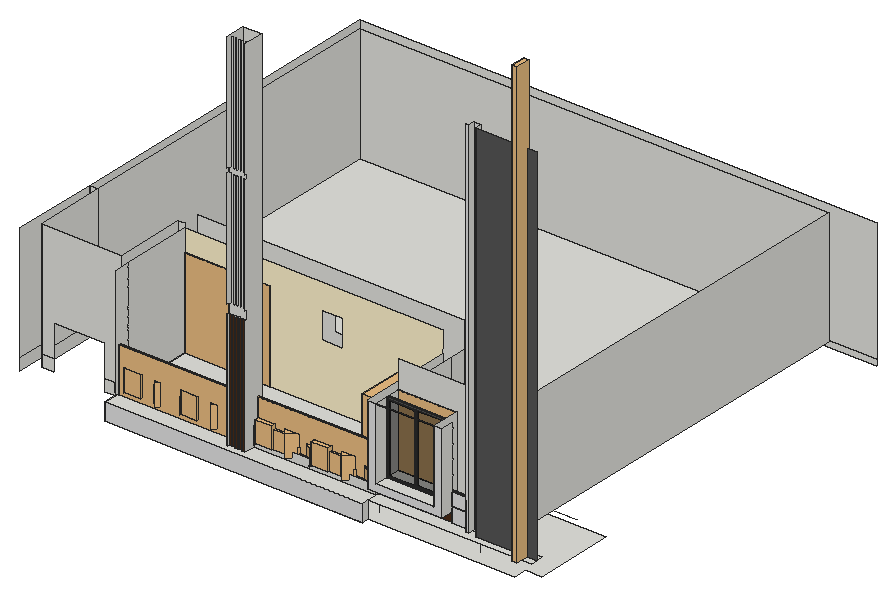
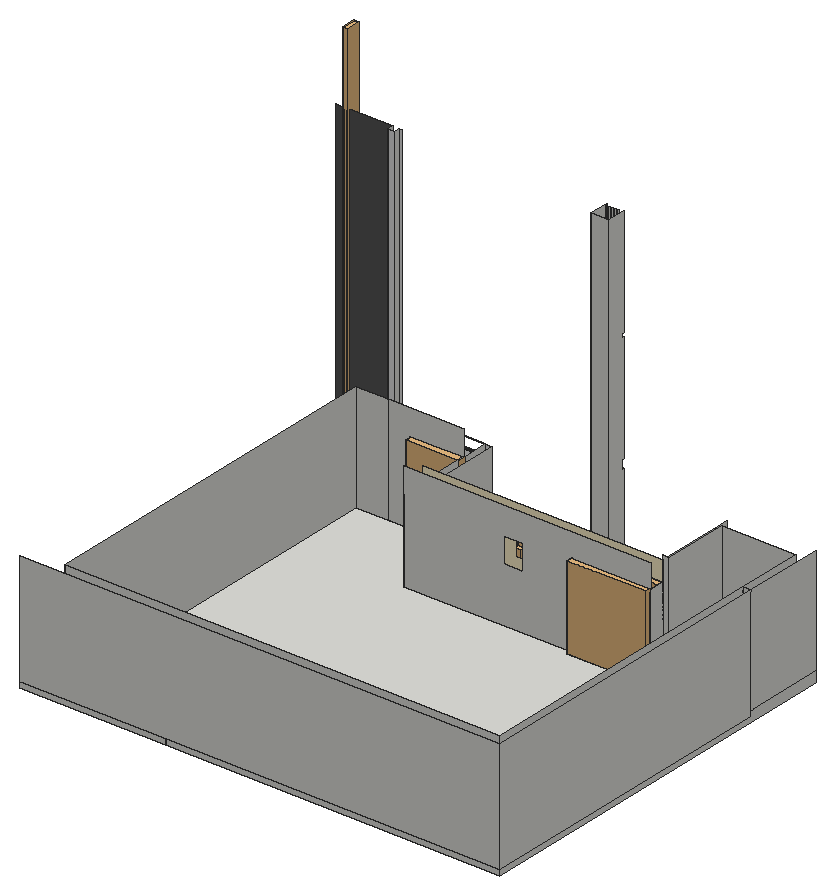
# SketchUp Ruby script. Lengths in inches.
U = 1.inch
M = Sketchup.active_model
def pt(a) = Geom::Point3d.new(a.map { |v| v * U })
def face(e, loops, mat)
  f = e.add_face(loops[0].map { |a| pt(a) })
  loops[1..].each { |l| e.add_face(l.map { |a| pt(a) }).erase! }
  f.material = f.back_material = mat if mat
  f
end
# faces: each face lists its corners as indices into pts; further lists are holes
def faces(e, pts, list, mat = nil) = list.each { |f| face(e, (f[0].is_a?(Array) ? f : [f]).map { |l| l.map { |i| pts[i] } }, mat) }
# xy, xz, yz: faces in a plane at the given z, y or x. An outline is a flat list of corners, or four numbers for a rectangle; further outlines are holes
def ring(l) = l.size == 4 ? [[l[0], l[1]], [l[2], l[1]], [l[2], l[3]], [l[0], l[3]]] : l.each_slice(2).to_a
def flat(e, list, mat, &to3) = list.each { |f| face(e, (f[0].is_a?(Array) ? f : [f]).map { |l| ring(l).map { |u, v| to3.(u, v) } }, mat) }
def xy(e, z, list, mat = nil) = flat(e, list, mat) { |x, y| [x, y, z] }
def xz(e, y, list, mat = nil) = flat(e, list, mat) { |x, z| [x, y, z] }
def yz(e, x, list, mat = nil) = flat(e, list, mat) { |y, z| [x, y, z] }
def lines(e, pts, list) = list.each { |a, b| e.add_line(pt(pts[a]), pt(pts[b])) }
# prism: a flat outline (further loops are holes) pulled along v
def prism(e, loops, v, mat = nil)
  f = face(e, loops, mat); d = Geom::Vector3d.new(v.map { |x| x * U })
  f.pushpull(f.normal.samedirection?(d) ? d.length : -d.length)
end
def box(e, o, s, mat = nil) = prism(e, [[o, [o[0] + s[0], o[1], o[2]], [o[0] + s[0], o[1] + s[1], o[2]], [o[0], o[1] + s[1], o[2]]]], [0, 0, s[2]], mat)
def at(x, y, z, deg = 0) = Geom::Transformation.translation(pt([x, y, z])) * Geom::Transformation.rotation(ORIGIN, Z_AXIS, deg.degrees)
def axes(o, x, y, z) = Geom::Transformation.new([*x, 0, *y, 0, *z, 0, *pt(o).to_a, 1])
def part(name) = M.definitions.add(name)
# library, detail: a bought-in or finely detailed component or shape, given as its bounding box
def library(name, o, s) = part(name).tap { |d| box(d.entities, o, s) }
def detail(e, o, s) = box(e.add_group.entities, o, s)
def put(e, d, t, mat = nil) = e.add_instance(d, t).tap { |i| i.material = mat if mat }
def group(e, t, mat = nil) = e.add_group.tap { |g| g.transformation = t; g.material = mat if mat }.entities
root = M.entities
M.materials.add("Glass_Tinted_Gray").color = [0, 0, 0]
M.materials["Glass_Tinted_Gray"].alpha = 0.125
M.materials.add("Material__1").color = [95, 70, 46]
M.materials.add("[0135_DarkGray]").color = [81, 81, 81]
M.materials.add("[Color D01]").color = [255, 242, 204]
M.materials.add("[Color M01]").color = [226, 226, 226]
M.materials.add("[Color M06]").color = [86, 86, 86]
M.materials.add("[Mirror 02]").color = [229, 229, 229]
M.materials.add("[Terrazzo Light Blue]").color = [196, 214, 227]
M.materials.add("[Wood Veneer 01]").color = [76, 44, 23]
c1 = library("Sliding Door",[0,0,0],[94.49,5.83,91.73])
c2 = part("glass-railing")
detail(c2.entities,[0,0,0],[1.26,75.59,33.1875])
c3 = library("Flora+17",[-57.52,158.6,-38.64],[66.99,62.88,77.28])
c4 = library("Group\#13",[-0.5,-0.5,0],[5.11,15.375,458.625])
c5 = library("Areca palm plant",[0,0,0],[49.1,36.6,54.46])
c6 = library("Group20\#1",[-20.81,-17.08,3.79],[39.86,39.43,37.51])
c7 = library("Group\#74",[-84.69,-90.07,-0.36],[176.51,175.13,171.4])
c8 = library("Group\#130",[-7.34,-1.2,0],[38.67,35.81,49.04])
c9 = library("Group38\#2",[14.01,28.44,-23.43],[18.58,18.32,38.89])
c10 = part("Group\#11")
put(c10.entities,c5,axes([-6.2,56.6,6.08],[0.45017,-0.56191,0],[0.66137,0.52986,0],[0,0,0.72]))
put(c10.entities,c5,axes([-6.2,158.41,6.08],[0.45017,-0.56191,0],[0.66137,0.52986,0],[0,0,0.72]))
put(c10.entities,c6,axes([18.97,181.79,4.77],[0,0.85,0],[-0.85,0,0],[0,0,0.85]))
put(c10.entities,c7,axes([14.93,71.3,6.05],[-0.04961,-0.08593,0],[0.08593,-0.04961,0],[0,0,0.10522]))
put(c10.entities,c7,axes([14.93,91.37,6.05],[-0.04961,-0.08593,0],[0.08593,-0.04961,0],[0,0,0.10522]))
put(c10.entities,c6,axes([18.97,79.98,4.77],[0,0.85,0],[-0.85,0,0],[0,0,0.85]))
put(c10.entities,c8,axes([24.9375,191.72,8],[0,0.79,0],[-0.79,0,0],[0,0,0.79]))
put(c10.entities,c7,axes([17.19,223.04,6.07],[-0.08133,-0.14087,0],[0.14087,-0.08133,0],[0,0,0.1725]))
put(c10.entities,c8,axes([24.9375,89.91,8],[0,0.79,0],[-0.79,0,0],[0,0,0.79]))
put(c10.entities,c7,axes([14.93,44.05,6.05],[-0.04961,-0.08593,0],[0.08593,-0.04961,0],[0,0,0.10522]))
put(c10.entities,c7,axes([14.93,145.87,6.05],[-0.04961,-0.08593,0],[0.08593,-0.04961,0],[0,0,0.10522]))
put(c10.entities,c9,axes([-4.1,100.66,28.17],[0.8848,0,0],[0,0.94674,0],[0,0,0.85826]))
put(c10.entities,c7,axes([14.93,173.12,6.05],[-0.04961,-0.08593,0],[0.08593,-0.04961,0],[0,0,0.10522]))
put(c10.entities,c9,axes([-4.1,-1.15,28.17],[0.8848,0,0],[0,0.94674,0],[0,0,0.85826]))
put(c10.entities,c7,axes([17.19,121.23,6.07],[-0.08133,-0.14087,0],[0.14087,-0.08133,0],[0,0,0.1725]))
put(c10.entities,c7,axes([14.93,193.18,6.05],[-0.04961,-0.08593,0],[0.08593,-0.04961,0],[0,0,0.10522]))
put(c10.entities,c7,axes([17.19,15.79,6.07],[-0.08133,-0.14087,0],[0.14087,-0.08133,0],[0,0,0.1725]))
g1 = group(c10.entities,at(0,0,0))
xy(g1,0,[[0,0,6,234.8],[30,0,36,234.8]])
xy(g1,3,[[6,0,30,234.8]])
xy(g1,7,[[6,5,30,229.8]],"Material__1")
xy(g1,15,[[[0,0,36,234.8],[6,5,30,229.8]]])
xz(g1,0,[[0,0,6,0,6,3,30,3,30,0,36,0,36,15,0,15]])
xz(g1,5,[[6,7,30,15]])
xz(g1,229.8,[[6,7,30,15]])
xz(g1,234.8,[[0,0,0,15,36,15,36,0,30,0,30,3,6,3,6,0]])
yz(g1,0,[[0,0,234.8,15]])
yz(g1,6,[[0,0,234.8,3],[5,7,229.8,15]])
yz(g1,30,[[0,0,234.8,3],[5,7,229.8,15]])
yz(g1,36,[[0,0,234.8,15]])
c11 = library("Curtains",[0,0,0],[121.73,8.19,117.22])
c12 = part("PENTEK_RP Fineline 50S_Sliding_DoorCase_E1")
box(c12.entities,[0,0,0],[1.51,3.66,99.27],"[0135_DarkGray]")
c13 = part("PENTEK_RP Fineline 50S_SlidingDooe_Case_E2")
box(c13.entities,[0,0,0],[96.25,3.66,1.51],"[0135_DarkGray]")
c14 = part("pentek_RP Fineline 50S_SlidingDoor_Case")
put(c14.entities,c12,at(97.76,0,0))
put(c14.entities,c13,at(1.51,0,0))
put(c14.entities,c12,at(0,0,0))
put(c14.entities,c13,at(1.51,0,97.76))
c15 = part("PENTEK_RP Fineline 50S_SlidingDoor_GlazingBead_2")
box(c15.entities,[0,0,0],[0.56,0.59,94.39],"[0135_DarkGray]")
c16 = part("PENTEK_RP Fineline 50S_SlidingDoor_Glass")
box(c16.entities,[0,0,0],[46.58,0.16,94.39],"Glass_Tinted_Gray")
c17 = part("PENTEK_RP Fineline 50S_SlidingDoor_GlazingBead")
box(c17.entities,[0,0,0],[45.47,0.59,0.56],"[0135_DarkGray]")
c18 = part("PENTEK_RP Fineline 50S_SlidingDoor_Leaf_E1")
xy(c18.entities,0,[[0,0,0.93,1.97],[0.93,1.57,1.49,1.97]],"[0135_DarkGray]")
xy(c18.entities,96.25,[[0,0,0.93,0,0.93,1.57,1.49,1.57,1.49,1.97,0,1.97]],"[0135_DarkGray]")
xz(c18.entities,0,[[0,0,0.93,96.25]],"[0135_DarkGray]")
xz(c18.entities,1.57,[[0.93,0,1.49,95.32],[0.93,95.32,1.49,96.25]],"[0135_DarkGray]")
xz(c18.entities,1.97,[[0,0,1.49,96.25]],"[0135_DarkGray]")
yz(c18.entities,0,[[0,0,1.97,96.25]],"[0135_DarkGray]")
yz(c18.entities,0.93,[[0,0,1.57,0.93],[0,0.93,1.57,95.32],[0,95.32,1.57,96.25]],"[0135_DarkGray]")
yz(c18.entities,1.49,[[1.57,0,1.97,95.32],[1.57,95.32,1.97,96.25]],"[0135_DarkGray]")
c19 = part("PENTEK_RP Fineline 50S_SlidingDoor_Leaf_E2")
xy(c19.entities,0,[[0,0,0,1.57,0.56,1.57,0.56,1.97,46.02,1.97,46.02,1.57,46.58,1.57,46.58,0]],"[0135_DarkGray]")
xy(c19.entities,0.93,[[0,0,46.58,1.57]],"[0135_DarkGray]")
xy(c19.entities,1.49,[[0.56,1.57,46.02,1.97]],"[0135_DarkGray]")
xz(c19.entities,0,[[0,0,46.58,0.93]],"[0135_DarkGray]")
xz(c19.entities,1.57,[[0,0,0.56,0.93],[46.02,0,46.58,0.93],[0.56,0.93,46.02,1.49]],"[0135_DarkGray]")
xz(c19.entities,1.97,[[0.56,0,46.02,1.49]],"[0135_DarkGray]")
yz(c19.entities,0,[[0,0,1.57,0.93]],"[0135_DarkGray]")
yz(c19.entities,0.56,[[1.57,0,1.97,0.93],[1.57,0.93,1.97,1.49]],"[0135_DarkGray]")
yz(c19.entities,46.02,[[1.57,0,1.97,0.93],[1.57,0.93,1.97,1.49]],"[0135_DarkGray]")
yz(c19.entities,46.58,[[0,0,1.57,0.93]],"[0135_DarkGray]")
c20 = part("PENTEK_RP Fineline S_SlidingDoor_Leaf1")
put(c20.entities,c15,at(0.93,0,0.93))
put(c20.entities,c15,at(46.96,0,0.93))
put(c20.entities,c16,at(1.49,1.42,0.93))
put(c20.entities,c17,at(1.49,0,0.93))
put(c20.entities,c16,at(1.49,0.59,0.93),"[Terrazzo Light Blue]")
put(c20.entities,c18,at(0,0,0))
put(c20.entities,c18,axes([48.44,0,0],[-1,0,0],[0,1,0],[0,0,1]))
put(c20.entities,c19,axes([0.93,0,96.25],[1,0,0],[0,1,0],[0,0,-1]))
put(c20.entities,c19,at(0.93,0,0))
put(c20.entities,c17,at(1.49,0,94.77))
c21 = part("PENTEK_RP Fineline 50S_SlidingDoor_Leaf2")
put(c21.entities,c16,at(1.49,1.42,0.93))
put(c21.entities,c17,at(1.49,0,94.77))
put(c21.entities,c15,at(46.96,0,0.93))
put(c21.entities,c16,at(1.49,0.59,0.93),"[Mirror 02]")
put(c21.entities,c15,at(0.93,0,0.93))
put(c21.entities,c18,at(0,0,0))
put(c21.entities,c18,axes([48.44,0,0],[-1,0,0],[0,1,0],[0,0,1]))
put(c21.entities,c17,at(1.49,0,0.93))
put(c21.entities,c19,axes([0.93,0,96.25],[1,0,0],[0,1,0],[0,0,-1]))
put(c21.entities,c19,at(0.93,0,0))
c22 = part("PENTEK - Slimmest Steel Sliding Door / Window\#1")
put(c22.entities,c14,at(0,-1.88,-0.09))
put(c22.entities,c20,at(1.51,-2.27,1.42))
put(c22.entities,c21,at(49.32,-0.3,1.42))
xy(root,120.375,[[[390.34,242.18,390.34,345.71,825.43,345.71,825.43,263.24,808.1,263.24,808.1,249.36,657.02,249.36,657.02,242.18],[608.73,281.66,610.52,281.89,612.18,282.58,613.6,283.67,614.7,285.1,615.39,286.76,615.62,288.54,615.39,290.33,614.7,291.99,613.6,293.42,612.18,294.51,610.52,295.2,608.73,295.43,606.95,295.2,605.29,294.51,603.86,293.42,602.77,291.99,602.08,290.33,601.84,288.54,602.08,286.76,602.77,285.1,603.86,283.67,605.29,282.58,606.95,281.89],[772.67,281.66,774.45,281.89,776.12,282.58,777.54,283.67,778.64,285.1,779.33,286.76,779.56,288.54,779.33,290.33,778.64,291.99,777.54,293.42,776.12,294.51,774.45,295.2,772.67,295.43,770.89,295.2,769.23,294.51,767.8,293.42,766.7,291.99,766.02,290.33,765.78,288.54,766.02,286.76,766.7,285.1,767.8,283.67,769.23,282.58,770.89,281.89],[432.89,282.54,434.44,282.75,435.89,283.35,437.13,284.3,438.08,285.54,438.68,286.99,438.89,288.54,438.68,290.1,438.08,291.54,437.13,292.79,435.89,293.74,434.44,294.34,432.89,294.54,431.34,294.34,429.89,293.74,428.65,292.79,427.69,291.54,427.09,290.1,426.89,288.54,427.09,286.99,427.69,285.54,428.65,284.3,429.89,283.35,431.34,282.75]],[657.02,242.18,657.09,249.36]])
xy(root,121.1875,[[608.73,281.66,606.95,281.89,605.29,282.58,603.86,283.67,602.77,285.1,602.08,286.76,601.84,288.54,602.08,290.33,602.77,291.99,603.86,293.42,605.29,294.51,606.95,295.2,608.73,295.43,610.52,295.2,612.18,294.51,613.6,293.42,614.7,291.99,615.39,290.33,615.62,288.54,615.39,286.76,614.7,285.1,613.6,283.67,612.18,282.58,610.52,281.89],[772.67,281.66,770.89,281.89,769.23,282.58,767.8,283.67,766.7,285.1,766.02,286.76,765.78,288.54,766.02,290.33,766.7,291.99,767.8,293.42,769.23,294.51,770.89,295.2,772.67,295.43,774.45,295.2,776.12,294.51,777.54,293.42,778.64,291.99,779.33,290.33,779.56,288.54,779.33,286.76,778.64,285.1,777.54,283.67,776.12,282.58,774.45,281.89],[432.89,282.54,431.34,282.75,429.89,283.35,428.65,284.3,427.69,285.54,427.09,286.99,426.89,288.54,427.09,290.1,427.69,291.54,428.65,292.79,429.89,293.74,431.34,294.34,432.89,294.54,434.44,294.34,435.89,293.74,437.13,292.79,438.08,291.54,438.68,290.1,438.89,288.54,438.68,286.99,438.08,285.54,437.13,284.3,435.89,283.35,434.44,282.75]])
xy(root,132,[[292.06,345.71,301.28,345.71,301.28,685.21,655.02,685.21,655.02,358.66,383.72,358.66,383.72,345.71,664.24,345.71,664.24,694.43,292.06,694.43],[301.28,345.71,301.28,685.21,655.02,685.21,655.02,358.66,383.72,358.66,383.72,345.71]])
xy(root,138,[[[390.34,242.18,657.02,242.18,657.02,249.36,657.09,249.36,657.09,345.71,478.4,345.71,478.4,362.65,390.9,362.65,390.9,345.71,390.34,345.71],[511.65,248.63,511.65,269.63,530.65,269.63,530.65,248.63,529.78,248.63,529.78,250.63,529.24,250.63,529.24,249.32,526.41,249.32,526.41,250.63,525.77,250.63,525.77,249.76,522.9375,249.76,522.9375,250.63,522.3,250.63,522.3,249.76,519.47,249.76,519.47,250.63,518.83,250.63,518.83,249.76,516,249.76,516,250.63,515.36,250.63,515.36,249.76,512.53,249.76,512.53,248.63]],[657.02,242.18,657.09,249.36],[657.09,249.36,825.43,249.36,825.43,256.61,814.72,256.61,814.72,258.49,811.07,258.49,811.07,256.61,761.98,256.61,761.98,263.24,657.09,263.24],[761.98,256.61,811.07,256.61,811.07,258.49,814.72,258.49,814.72,256.61,825.43,256.61,825.43,263.24,761.98,263.24],[665.11,279.2,784.56,279.2,784.56,683.75,301.28,683.75,301.28,345.71,390.34,345.71,390.34,362.65,665.11,362.65],
  [390.34,345.71,390.9,362.65]])
xy(root,138.38,[[751.93,256.61,754.62,263.24],[733.09,261.68,751.93,263.24]])
xy(root,147.96,[[657.09,249.36,733.09,263.24]])
xy(root,152.68,[[733.09,261.68,751.93,263.24]])
xy(root,153.62,[[733.09,261.68,751.93,263.24]])
xy(root,155.18,[[664.71,249.36,724.59,279.2],[664.71,279.2,665.11,345.71],[665.11,279.2,665.59,345.71]])
xy(root,166.98,[[733.09,261.68,751.93,263.24]])
xz(root,242.18,[[657.02,120.375,657.09,138]])
xz(root,242.18,[[390.34,120.375,657.02,138]],"[Color M01]")
xz(root,248.63,[[511.65,138,512.53,259.25],[529.78,138,530.65,259.25]])
xz(root,249.32,[[526.41,138,529.24,259.25]],"[Wood Veneer 01]")
xz(root,249.36,[[657.02,120.375,657.09,138]])
xz(root,249.36,[[[657.09,147.96,733.09,147.96,733.09,230.43,732.65,230.43,732.65,229.99,657.09,229.99],[664.71,155.18,724.59,229.87]]],"[Color M01]")
xz(root,249.76,[[512.53,138,515.36,259.25],[516,138,518.83,259.25],[519.47,138,522.3,259.25],[522.9375,138,525.77,259.25]],"[Wood Veneer 01]")
xz(root,250.63,[[[515.36,138,516,138,516,259.25,518.83,259.25,518.83,138,519.47,138,519.47,259.25,522.3,259.25,522.3,138,522.9375,138,522.9375,259.25,525.77,259.25,525.77,138,526.41,138,526.41,259.25,529.24,259.25,529.24,138,529.78,138,529.78,259.25,530.65,259.25,530.65,268.625,529.78,268.625,529.78,389.875,530.65,389.875,530.65,394.625,529.78,394.625,529.78,515.875,529.24,515.875,529.24,394.625,526.41,394.625,526.41,515.875,525.77,515.875,525.77,394.625,522.9375,394.625,522.9375,515.875,522.3,515.875,522.3,394.625,519.47,394.625,519.47,515.875,518.83,515.875,518.83,394.625,516,394.625,516,515.875,515.36,515.875,515.36,394.625,511.65,394.625,511.65,389.875,515.36,389.875,515.36,268.625,511.65,268.625,511.65,259.25,515.36,259.25],[516,268.625,518.83,389.875],[519.47,268.625,522.3,389.875],[526.41,268.625,529.24,389.875],[522.9375,268.625,525.77,389.875]]])
xz(root,256.61,[[751.93,138.38,754.62,515.875]],"[Color M01]")
xz(root,256.61,[[761.98,138,811.07,515.875],[814.72,138,825.43,515.875]],"[Color M06]")
xz(root,261.68,[[733.09,138.38,751.93,152.68],[733.09,153.62,751.93,166.98]],"[Color M01]")
xz(root,263.24,[[733.09,152.68,751.93,153.62],[733.09,166.98,751.93,167.92]])
xz(root,263.24,[[754.62,138,761.98,515.875]],"[Color M01]")
xz(root,263.24,[[657.09,138,754.62,138,754.62,138.38,733.09,138.38,733.09,147.96,657.09,147.96]],"[Wood Veneer 01]")
xz(root,269.63,[[511.65,138,530.65,515.875]])
xz(root,272.46,[[301.28,126,314.4,138],[366.4,126,383.72,138],[301.28,138,301.28,258,383.72,258,383.72,138,366.4,138,366.4,171.49,314.4,171.49,314.4,138]])
xz(root,279.2,[[665.11,138,665.11,155.18,724.59,155.18,724.59,229.87,665.11,229.87,665.11,258,749.59,258,749.59,138],[749.59,138,784.56,258],[664.71,155.18,665.59,229.87]])
xz(root,345.71,[[390.34,120.375,655.02,126],[655.02,120.375,664.24,126],[390.34,126,655.02,132],[655.02,126,664.24,132],[292.06,132,301.28,138],
  [301.28,132,383.72,138],[383.72,132,390.34,138],[292.06,138,301.28,258],[383.72,138,390.34,258],[390.34,138,390.9,231.125],
  [664.71,155.18,665.11,229.87],[665.11,155.18,665.59,229.87]])
xz(root,345.71,[[[478.4,138,657.09,138,657.09,230.43,655.52,230.43,655.52,235.64,657.09,235.64,657.09,253.375,390.34,253.375,390.34,231.125,478.4,231.125],[531.79,199.5625,553.72,227.9375]]],"[Color D01]")
xz(root,358.66,[[383.72,126,655.02,132]])
xz(root,362.65,[[390.34,138,390.9,231.125],[[478.4,138,478.4,231.125,390.34,231.125,390.34,258,665.11,258,665.11,138],[531.79,199.5625,553.72,227.9375]]])
xz(root,683.75,[[301.28,138,784.56,258]])
xz(root,685.21,[[301.28,126,655.02,132]])
xz(root,694.43,[[292.06,126,664.24,132],[664.24,126,825.43,132],[292.06,132,825.43,258]])
yz(root,292.06,[[256.61,126,256.61,138,345.71,138,345.71,132,694.43,132,694.43,126],[345.71,132,694.43,258],[256.61,138,345.71,258]])
yz(root,301.28,[[272.46,126,685.21,126,685.21,132,345.71,132,345.71,138,272.46,138],[272.46,138,345.71,258],[345.71,138,683.75,258]])
yz(root,383.72,[[272.46,126,272.46,138,345.71,138,345.71,132,358.66,132,358.66,126],[272.46,138,345.71,258]])
yz(root,390.34,[[242.18,120.375,256.61,126],[256.61,120.375,272.46,126],[272.46,120.375,345.71,126],[242.18,126,256.61,138],[256.61,126,272.46,138],
  [272.46,126,345.71,138],[256.61,138,272.46,253.375],[272.46,138,345.71,253.375],[345.71,138,362.65,231.125]])
yz(root,390.9,[[345.71,138,362.65,231.125]])
yz(root,478.4,[[345.71,138,362.65,231.125]])
yz(root,511.65,[[248.63,138,248.63,259.25,250.63,259.25,250.63,268.625,248.63,268.625,248.63,389.875,250.63,389.875,250.63,394.625,248.63,394.625,248.63,515.875,269.63,515.875,269.63,138]])
yz(root,512.53,[[248.63,138,249.76,259.25]])
yz(root,515.36,[[249.76,138,250.63,259.25]])
yz(root,516,[[249.76,138,250.63,259.25]])
yz(root,518.83,[[249.76,138,250.63,259.25]])
yz(root,519.47,[[249.76,138,250.63,259.25]])
yz(root,522.3,[[249.76,138,250.63,259.25]])
yz(root,522.9375,[[249.76,138,250.63,259.25]])
yz(root,525.77,[[249.76,138,250.63,259.25]])
yz(root,526.41,[[249.32,138,250.63,259.25]])
yz(root,529.24,[[249.32,138,250.63,259.25]])
yz(root,529.78,[[248.63,138,250.63,259.25]])
yz(root,530.65,[[248.63,138,269.63,138,269.63,515.875,248.63,515.875,248.63,394.625,250.63,394.625,250.63,389.875,248.63,389.875,248.63,268.625,250.63,268.625,250.63,259.25,248.63,259.25]])
yz(root,655.02,[[358.66,126,685.21,132]])
yz(root,657.02,[[242.18,120.375,249.36,138]])
yz(root,657.09,[[242.18,120.375,249.36,138],[263.24,138,263.24,147.96,249.36,147.96,249.36,230.43,345.71,230.43,345.71,138]])
yz(root,664.24,[[345.71,126,694.43,132]])
yz(root,664.71,[[249.36,155.18,279.2,229.87]])
yz(root,665.11,[[279.2,138,345.71,155.18],[345.71,138,362.65,155.18],[345.71,155.18,362.65,229.87]])
yz(root,665.59,[[279.2,155.18,345.71,229.87]])
yz(root,724.59,[[249.36,155.18,279.2,229.87]])
yz(root,733.09,[[261.68,138.38,263.24,147.96],[249.36,147.96,261.68,147.96,261.68,152.68,263.24,152.68,263.24,153.62,261.68,153.62,261.68,166.98,263.24,166.98,263.24,167.92,261.68,167.92,261.68,181.28,263.24,181.28,263.24,182.22,261.68,182.22,261.68,195.58,263.24,195.58,263.24,196.52,261.68,196.52,261.68,209.875,263.24,209.875,263.24,210.8125,261.68,210.8125,261.68,224.18,263.24,224.18,263.24,225.11,261.68,225.11,261.68,230.43,249.36,230.43],[261.68,147.96,263.24,152.68],[261.68,153.62,263.24,166.98]])
yz(root,751.93,[[256.61,138.38,261.68,147.96],[256.61,147.96,261.68,152.68],[256.61,152.68,263.24,153.62],[256.61,153.62,261.68,166.98],[256.61,166.98,263.24,167.92]])
yz(root,754.62,[[256.61,138.38,263.24,515.875]])
yz(root,761.98,[[256.61,138,263.24,515.875]])
yz(root,784.56,[[279.2,138,683.75,258]])
yz(root,811.07,[[256.61,138,258.49,515.875]])
yz(root,814.72,[[256.61,138,258.49,515.875]])
p = [[606.95,281.89,121.1875],[608.73,281.66,121.1875],[608.73,281.66,120.375],[606.95,281.89,120.375],[610.52,281.89,121.1875],[610.52,281.89,120.375],
  [770.89,281.89,121.1875],[772.67,281.66,121.1875],[772.67,281.66,120.375],[770.89,281.89,120.375],[774.45,281.89,121.1875],[774.45,281.89,120.375],
  [605.29,282.58,121.1875],[605.29,282.58,120.375],[612.18,282.58,121.1875],[612.18,282.58,120.375],[769.23,282.58,121.1875],[769.23,282.58,120.375],
  [776.12,282.58,121.1875],[776.12,282.58,120.375],[431.34,282.75,121.1875],[432.89,282.54,121.1875],[432.89,282.54,120.375],[431.34,282.75,120.375],
  [434.44,282.75,121.1875],[434.44,282.75,120.375],[603.86,283.67,121.1875],[603.86,283.67,120.375],[613.6,283.67,121.1875],[613.6,283.67,120.375],
  [767.8,283.67,121.1875],[767.8,283.67,120.375],[777.54,283.67,121.1875],[777.54,283.67,120.375],[429.89,283.35,121.1875],[429.89,283.35,120.375],
  [435.89,283.35,121.1875],[435.89,283.35,120.375],[428.65,284.3,121.1875],[428.65,284.3,120.375],[437.13,284.3,121.1875],[437.13,284.3,120.375],
  [602.77,285.1,121.1875],[602.77,285.1,120.375],[614.7,285.1,121.1875],[614.7,285.1,120.375],[766.7,285.1,121.1875],[766.7,285.1,120.375],
  [778.64,285.1,121.1875],[778.64,285.1,120.375],[427.69,285.54,121.1875],[427.69,285.54,120.375],[438.08,285.54,121.1875],[438.08,285.54,120.375],
  [602.08,286.76,121.1875],[602.08,286.76,120.375],[615.39,286.76,121.1875],[615.39,286.76,120.375],[766.02,286.76,121.1875],[766.02,286.76,120.375],
  [779.33,286.76,121.1875],[779.33,286.76,120.375],[427.09,286.99,121.1875],[427.09,286.99,120.375],[438.68,286.99,121.1875],[438.68,286.99,120.375],
  [601.84,288.54,121.1875],[601.84,288.54,120.375],[615.62,288.54,121.1875],[615.62,288.54,120.375],[765.78,288.54,121.1875],[765.78,288.54,120.375],
  [779.56,288.54,121.1875],[779.56,288.54,120.375],[426.89,288.54,121.1875],[426.89,288.54,120.375],[438.89,288.54,121.1875],[438.89,288.54,120.375],
  [427.09,290.1,121.1875],[427.09,290.1,120.375],[438.68,290.1,121.1875],[438.68,290.1,120.375],[602.08,290.33,121.1875],[602.08,290.33,120.375],
  [615.39,290.33,121.1875],[615.39,290.33,120.375],[766.02,290.33,121.1875],[766.02,290.33,120.375],[779.33,290.33,121.1875],[779.33,290.33,120.375],
  [427.69,291.54,121.1875],[427.69,291.54,120.375],[438.08,291.54,121.1875],[438.08,291.54,120.375],[602.77,291.99,121.1875],[602.77,291.99,120.375],
  [614.7,291.99,121.1875],[614.7,291.99,120.375],[766.7,291.99,121.1875],[766.7,291.99,120.375],[778.64,291.99,121.1875],[778.64,291.99,120.375],
  [428.65,292.79,121.1875],[428.65,292.79,120.375],[437.13,292.79,121.1875],[437.13,292.79,120.375],[603.86,293.42,121.1875],[603.86,293.42,120.375],
  [613.6,293.42,121.1875],[613.6,293.42,120.375],[767.8,293.42,121.1875],[767.8,293.42,120.375],[777.54,293.42,121.1875],[777.54,293.42,120.375],
  [429.89,293.74,121.1875],[429.89,293.74,120.375],[435.89,293.74,121.1875],[435.89,293.74,120.375],[605.29,294.51,121.1875],[605.29,294.51,120.375],
  [612.18,294.51,121.1875],[612.18,294.51,120.375],[769.23,294.51,121.1875],[769.23,294.51,120.375],[776.12,294.51,121.1875],[776.12,294.51,120.375],
  [431.34,294.34,121.1875],[431.34,294.34,120.375],[434.44,294.34,121.1875],[434.44,294.34,120.375],[432.89,294.54,121.1875],[432.89,294.54,120.375],
  [606.95,295.2,121.1875],[606.95,295.2,120.375],[610.52,295.2,121.1875],[610.52,295.2,120.375],[770.89,295.2,121.1875],[770.89,295.2,120.375],
  [774.45,295.2,121.1875],[774.45,295.2,120.375],[608.73,295.43,121.1875],[608.73,295.43,120.375],[772.67,295.43,121.1875],[772.67,295.43,120.375],
  [664.24,345.71,126],[795.31,345.71,126],[761.98,263.24,120.375],[761.98,263.24,138],[657.09,263.24,138],[657.09,263.24,120.375]]
faces(root,p,[[0,1,2,3],[1,4,5,2],[6,7,8,9],[7,10,11,8],[12,0,3,13],[4,14,15,5],[16,6,9,17],[10,18,19,11],
  [20,21,22,23],[21,24,25,22],[26,12,13,27],[14,28,29,15],[30,16,17,31],[18,32,33,19],[34,20,23,35],[24,36,37,25],
  [38,34,35,39],[36,40,41,37],[42,26,27,43],[28,44,45,29],[46,30,31,47],[32,48,49,33],[50,38,39,51],[40,52,53,41],
  [54,42,43,55],[44,56,57,45],[58,46,47,59],[48,60,61,49],[62,50,51,63],[52,64,65,53],[66,54,55,67],[56,68,69,57],
  [70,58,59,71],[60,72,73,61],[74,62,63,75],[64,76,77,65],[78,74,75,79],[76,80,81,77],[82,66,67,83],[68,84,85,69],
  [86,70,71,87],[72,88,89,73],[90,78,79,91],[80,92,93,81],[94,82,83,95],[84,96,97,85],[98,86,87,99],[88,100,101,89],
  [102,90,91,103],[92,104,105,93],[106,94,95,107],[96,108,109,97],[110,98,99,111],[100,112,113,101],[114,102,103,115],[104,116,117,105],
  [118,106,107,119],[108,120,121,109],[122,110,111,123],[112,124,125,113],[126,114,115,127],[116,128,129,117],[130,126,127,131],[128,130,131,129],
  [132,118,119,133],[120,134,135,121],[136,122,123,137],[124,138,139,125],[140,132,133,141],[134,140,141,135],[142,136,137,143],[138,142,143,139]])
lines(root,p,[[144,145],[146,147],[148,149]])
put(root,c1,axes([390.9,345.71,138],[0.92604,0,0],[0,1,0],[0,0,1.01518]))
put(root,c2,axes([532.09,264.86,138],[0,-1.29,0],[1.65356,0,0],[0,0,1.37437]))
put(root,c2,axes([391.78,261.07,138],[0,-1.29,0],[1.60489,0,0],[0,0,1.38316]))
put(root,c3,axes([661.74,164.23,169.6875],[0.82,0,0],[0,0.82,0],[0,0,0.82]))
put(root,c4,at(810.6,244.11,138))
put(root,c10,axes([520.88,260.15,138],[0,0.57,0],[-0.57,0,0],[0,0,0.57]),"[Color M01]")
put(root,c10,axes([655.82,260.15,138],[0,0.57,0],[-0.57,0,0],[0,0,0.57]))
put(root,c11,axes([390.9,360.28,139.375],[0.71882,0,0],[0,1,0],[0,0,0.79]))
put(root,c22,axes([665.02,264.37,155.25],[0.6,0,0],[0,0.6,0],[0,0,0.7536]))
put(root,c11,axes([664.45,278.43,155.98],[0.4835,0,0],[0,1,0],[0,0,0.63137]))
